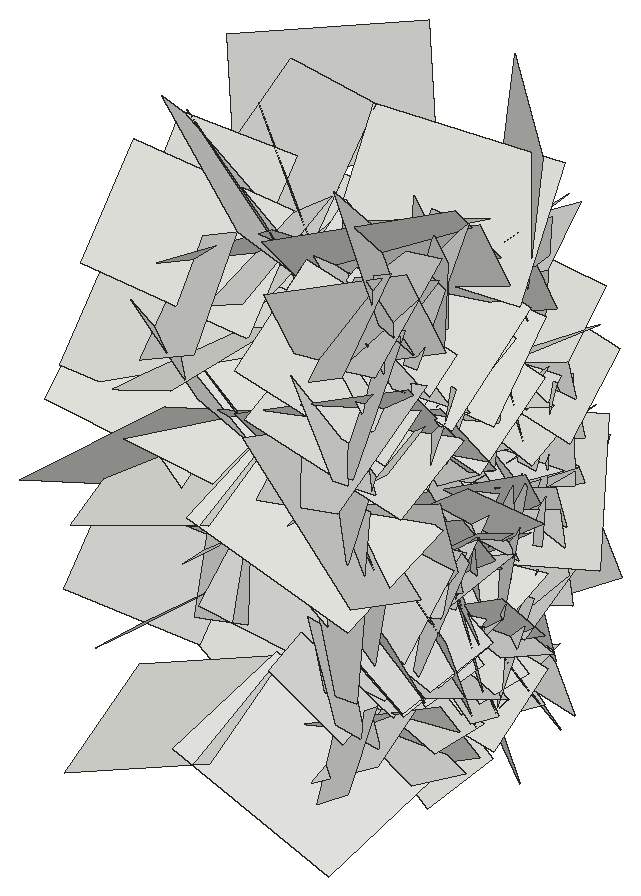
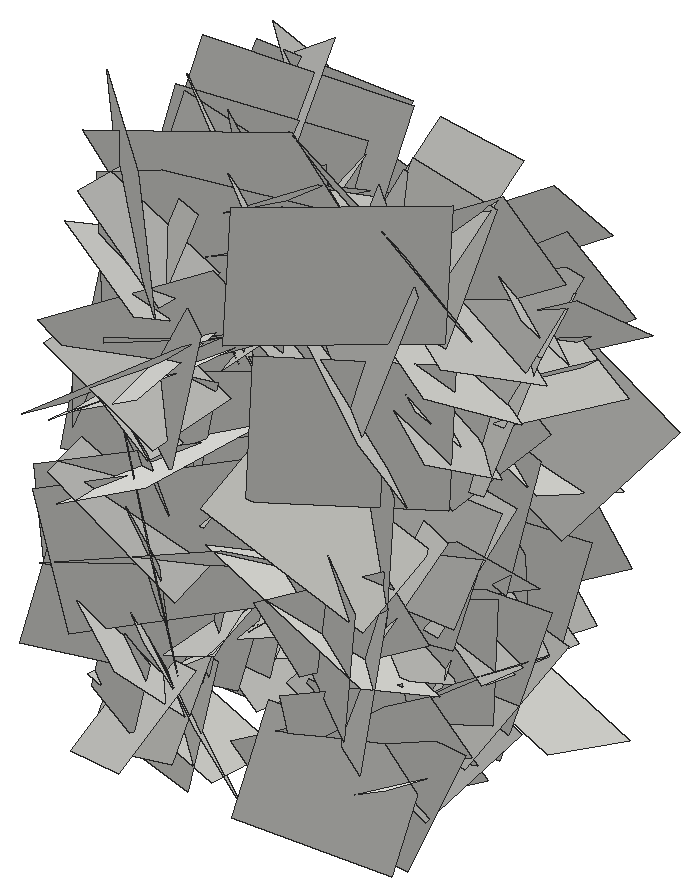
# SketchUp Ruby script. Lengths in inches.
U = 1.inch
M = Sketchup.active_model
def pt(a) = Geom::Point3d.new(a.map { |v| v * U })
def face(e, loops, mat)
  f = e.add_face(loops[0].map { |a| pt(a) })
  loops[1..].each { |l| e.add_face(l.map { |a| pt(a) }).erase! }
  f.material = f.back_material = mat if mat
  f
end
# faces: each face lists its corners as indices into pts; further lists are holes
def faces(e, pts, list, mat = nil) = list.each { |f| face(e, (f[0].is_a?(Array) ? f : [f]).map { |l| l.map { |i| pts[i] } }, mat) }
# xy, xz, yz: faces in a plane at the given z, y or x. An outline is a flat list of corners, or four numbers for a rectangle; further outlines are holes
def ring(l) = l.size == 4 ? [[l[0], l[1]], [l[2], l[1]], [l[2], l[3]], [l[0], l[3]]] : l.each_slice(2).to_a
def flat(e, list, mat, &to3) = list.each { |f| face(e, (f[0].is_a?(Array) ? f : [f]).map { |l| ring(l).map { |u, v| to3.(u, v) } }, mat) }
def xy(e, z, list, mat = nil) = flat(e, list, mat) { |x, y| [x, y, z] }
def xz(e, y, list, mat = nil) = flat(e, list, mat) { |x, z| [x, y, z] }
def yz(e, x, list, mat = nil) = flat(e, list, mat) { |y, z| [x, y, z] }
def lines(e, pts, list) = list.each { |a, b| e.add_line(pt(pts[a]), pt(pts[b])) }
# prism: a flat outline (further loops are holes) pulled along v
def prism(e, loops, v, mat = nil)
  f = face(e, loops, mat); d = Geom::Vector3d.new(v.map { |x| x * U })
  f.pushpull(f.normal.samedirection?(d) ? d.length : -d.length)
end
def box(e, o, s, mat = nil) = prism(e, [[o, [o[0] + s[0], o[1], o[2]], [o[0] + s[0], o[1] + s[1], o[2]], [o[0], o[1] + s[1], o[2]]]], [0, 0, s[2]], mat)
def at(x, y, z, deg = 0) = Geom::Transformation.translation(pt([x, y, z])) * Geom::Transformation.rotation(ORIGIN, Z_AXIS, deg.degrees)
def axes(o, x, y, z) = Geom::Transformation.new([*x, 0, *y, 0, *z, 0, *pt(o).to_a, 1])
def part(name) = M.definitions.add(name)
# library, detail: a bought-in or finely detailed component or shape, given as its bounding box
def library(name, o, s) = part(name).tap { |d| box(d.entities, o, s) }
def detail(e, o, s) = box(e.add_group.entities, o, s)
def put(e, d, t, mat = nil) = e.add_instance(d, t).tap { |i| i.material = mat if mat }
def group(e, t, mat = nil) = e.add_group.tap { |g| g.transformation = t; g.material = mat if mat }.entities
root = M.entities
c1 = part("Component\#6")
p = [[0.01,0,0],[0,3.24,4.54],[4.32,3.24,4.54],[4.33,0,0]]
faces(c1.entities,p,[[0,1,2,3]])
put(root,c1,axes([400.91,167.01,8.33],[0.18631,0.3359,0.73427],[0.04897,0.74605,-0.35235],[0.8545,-0.11599,-0.1399]))
put(root,c1,axes([400.91,166.18,19.56],[-0.12535,0.0531,1.28965],[-0.2192,1.27754,-0.07157],[1.35051,0.21229,0.10808]))
put(root,c1,axes([400.91,168.14,0.12],[-0.06773,-0.63363,0.78179],[0.11595,0.77435,0.63654],[1.06038,-0.12515,-0.01967]))
put(root,c1,axes([400.91,169.19,10.7],[-0.0913,0.46499,-1.24639],[-0.29576,-1.22753,-0.43867],[1.37875,-0.23253,-0.17663]))
put(root,c1,axes([404.88,165.96,10.85],[0.09912,0.20412,-0.70693],[0.02587,-0.71308,-0.20267],[-0.77953,0.00229,-0.09661]))
put(root,c1,axes([404.88,161.25,17.66],[0.25985,0.898,-0.37026],[0.14737,-0.41038,-0.90325],[-1.01902,0.16964,-0.22504]))
put(root,c1,axes([404.88,162.79,15.86],[0.07285,0.46729,0.4905],[-0.02436,0.49435,-0.46773],[-0.71769,0.03066,0.06566]))
put(root,c1,axes([400.91,167.22,15.375],[-0.0235,-0.92066,-0.53568],[-0.01768,-0.53543,0.92093],[1.12894,-0.02755,0.00327]))
put(root,c1,axes([400.91,167.28,17.92],[-0.19972,-0.96368,-0.57877],[0.14667,-0.60226,0.95775],[1.18251,-0.08806,-0.21655]))
put(root,c1,axes([400.91,157.18,19.73],[-0.07599,0.81527,0.8297],[-0.084,0.82592,-0.8184],[1.23014,0.10676,-0.00463]))
put(root,c1,axes([400.91,167.18,1.59],[-0.07507,-1.0991,0.32301],[-0.05871,0.32653,1.09895],[1.2129,-0.05222,0.07319]))
put(root,c1,axes([400.91,168.87,14.79],[0.03205,0.06087,-1.12787],[-0.16204,-1.11767,-0.06442],[1.18627,-0.15431,0.02167]))
put(root,c1,axes([400.91,166.01,11.8],[0.21466,0.53877,-0.68228],[-0.03009,-0.69607,-0.55809],[0.92102,-0.14831,0.14079]))
put(root,c1,axes([400.91,163.57,3.71],[0.11292,-0.2033,0.99476],[-0.09749,0.99417,0.21302],[1.07181,0.11185,-0.08542]))
put(root,c1,axes([400.91,159.91,9.22],[-0.2022,-1.20502,0.50539],[-0.1049,0.52261,1.20871],[1.38114,-0.13672,0.1658]))
put(root,c1,axes([400.91,162.44,14.8125],[-0.22172,-1.13603,-0.19278],[0.19013,-0.22565,1.13507],[1.20652,-0.17321,-0.21429]))
put(root,c1,axes([400.91,160.62,5.12],[0.08568,1.04485,0.18773],[-0.09569,0.19436,-1.04286],[1.1212,-0.06325,-0.10335]))
put(root,c1,axes([404.88,162.91,7.6875],[0.03517,0.6334,0.29771],[0.1292,0.28826,-0.62688],[-0.73053,0.08147,-0.09654]))
put(root,c1,axes([400.91,163.93,5.47],[0.11462,-1.01834,-0.26907],[-0.10191,-0.2789,1.0169],[1.11183,0.07941,0.12095]))
put(root,c1,axes([400.91,156.14,6.5],[0.17845,0.35117,0.84391],[0.01887,0.85668,-0.36003],[0.96872,-0.08137,-0.14844]))
put(root,c1,axes([404.88,170.02,6.34],[0.13634,-0.30577,-0.6303],[0.02329,-0.63876,0.31436],[-0.74222,-0.07621,-0.10592]))
put(root,c1,axes([400.91,160.14,4.78],[0.03826,-0.47304,0.81506],[0.18962,0.80427,0.45886],[0.98077,-0.13704,-0.12051]))
put(root,c1,axes([400.91,166.625,12.7],[0.17127,1.04033,-0.10676],[-0.13463,-0.08771,-1.04688],[1.10034,-0.17266,-0.11147]))
put(root,c1,axes([400.91,168.99,0.33],[0.20008,-0.71049,0.66963],[-0.07161,0.67089,0.73087],[1.03242,0.18422,-0.07908]))
put(root,c1,axes([400.91,164.18,5.53],[0.00871,-1.21515,-0.1589],[-0.11926,-0.15898,1.20995],[1.29354,-0.00648,0.11262]))
put(root,c1,axes([404.88,159.77,13.93],[0.14822,0.47929,0.38572],[-0.01533,0.39801,-0.48932],[-0.65196,0.0996,0.0992]))
put(root,c1,axes([400.91,165.6875,8.33],[0.14254,-0.77018,0.64298],[0.05856,0.65343,0.77114],[1.06187,0.06735,-0.12884]))
put(root,c1,axes([400.91,164.53,2.65],[0.11418,0.95876,0.15487],[0.16789,0.13639,-0.95453],[1.01568,-0.13033,0.14037]))
put(root,c1,axes([404.88,155.94,6.59],[0.14653,0.65267,0.04592],[0.0729,0.03218,-0.6644],[-0.6897,0.14207,-0.06047]))
put(root,c1,axes([400.91,170.79,17.67],[0.07972,-0.69903,-0.88266],[-0.01234,-0.88506,0.69994],[1.19343,0.03754,0.0662]))
put(root,c1,axes([400.91,165.97,13.03],[0.11695,-0.23373,1.15092],[-0.10796,1.14973,0.24325],[1.24018,0.12213,-0.08736]))
put(root,c1,axes([404.88,164.09,3.1],[0.16189,-0.51758,0.36968],[0.06161,0.38995,0.52196],[-0.67139,-0.08902,0.13704]))
put(root,c1,axes([400.91,155.93,16.01],[0.06166,0.77521,1.08886],[-0.24821,1.07895,-0.75564],[1.39492,0.15772,-0.18259]))
put(root,c1,axes([400.91,163.21,2.24],[-0.08398,-0.53221,1.10764],[0.11648,1.10243,0.53756],[1.29738,-0.13342,0.02343]))
put(root,c1,axes([400.91,161.02,12.77],[0.04866,0.36936,-1.04237],[0.12613,-1.03886,-0.36288],[1.16543,0.09701,0.0828]))
put(root,c1,axes([400.91,162.03,18.62],[0.15865,-0.78055,-0.79386],[-0.03617,-0.80384,0.78393],[1.17956,0.08034,0.13081]))
put(root,c1,axes([400.91,161.03,16.77],[-0.02327,0.73455,-0.90907],[0.17416,-0.89826,-0.72978],[1.22657,0.14148,0.08637]))
put(root,c1,axes([400.91,163.86,1.73],[0.03729,0.66749,1.03354],[-0.00972,1.03407,-0.66752],[1.30413,-0.01138,-0.03452]))
put(root,c1,axes([400.91,162.85,15.75],[0.04254,-1.00522,0.67204],[0.02385,0.67292,1.00519],[1.28151,0.02084,-0.04102]))
put(root,c1,axes([400.91,163.36,23.49],[0.04873,0.57368,-1.00395],[0.12423,-1.00188,-0.56714],[1.21936,0.07915,0.09791]))
put(root,c1,axes([400.91,159.69,18.96],[0.02704,0.74145,1.09535],[-0.09362,1.09406,-0.73853],[1.39894,0.05888,-0.07059]))
put(root,c1,axes([400.91,166.4,18.65],[-0.092,-1.19571,-0.63762],[0.0325,-0.6405,1.19693],[1.43603,-0.06211,-0.06794]))
put(root,c1,axes([400.91,155.03,14.95],[-0.10989,1.07322,0.82249],[0.07177,0.82799,-1.07186],[1.43147,0.04087,0.11688]))
put(root,c1,axes([400.91,159.14,18.38],[0.07521,0.79304,-0.86536],[0.12573,-0.86735,-0.78513],[1.23784,0.03991,0.13233]))
put(root,c1,axes([400.91,168.375,23.9],[-0.0952,-0.72561,-1.04974],[0.29336,-1.03837,0.69407],[1.32049,0.17837,-0.22987]))
put(root,c1,axes([400.91,157.93,15.34],[0.27083,1.19165,0.15594],[-0.0802,0.17506,-1.21378],[1.27139,-0.2428,-0.10978]))
put(root,c1,axes([400.91,162.31,11.53],[0.17206,0.75955,-0.87532],[0.12131,-0.89005,-0.75111],[1.22246,-0.01858,0.19774]))
put(root,c1,axes([400.91,165.1,2.71],[-0.06092,-1.21711,0.58199],[0.18306,0.57109,1.21136],[1.41828,-0.12599,-0.13136]))
put(root,c1,axes([400.91,170.58,10.37],[0.24309,-1.14649,0.14454],[0.04952,0.15643,1.16674],[1.2239,0.22139,-0.07591]))
put(root,c1,axes([400.91,161.07,7.88],[0.0926,0.91308,0.78861],[0.24837,0.76278,-0.90913],[1.25453,-0.21841,0.12178]))
put(root,c1,axes([400.91,171.01,11.29],[0.23144,-0.15428,-1.27652],[-0.01824,-1.29503,0.15357],[1.36284,0.00887,0.21884]))
put(root,c1,axes([400.91,167.61,21.95],[0.32344,0.31012,-1.26322],[-0.1451,-1.28265,-0.34796],[1.37111,-0.2089,0.26116]))
put(root,c1,axes([400.91,161.91,24.73],[0.20116,0.87735,-0.9177],[0.06395,-0.93308,-0.87958],[1.34427,-0.0869,0.17917]))
put(root,c1,axes([400.91,161.24,11.55],[0.08722,-1.18104,-0.51149],[0.30261,-0.48302,1.16122],[1.33028,0.18731,-0.23062]))
put(root,c1,axes([400.91,160.65,1.35],[0.1594,-1.22011,-0.46707],[0.28659,-0.43091,1.2127],[1.35486,0.2347,-0.20157]))
put(root,c1,axes([400.91,170.67,8.29],[0.13658,-1.14766,-0.62909],[0.33753,-0.58565,1.13362],[1.34561,0.26339,-0.2205]))
put(root,c1,axes([400.91,161.87,9.58],[0.35888,-0.49511,-1.17449],[0.11741,-1.19919,0.53746],[1.34594,0.23663,0.26628]))
put(root,c1,axes([414.68,161.87,9.58],[-0.35888,-0.49511,-1.17449],[-0.11741,-1.19919,0.53746],[-1.34594,0.23663,0.26628]))
put(root,c1,axes([414.68,170.67,8.29],[-0.13658,-1.14766,-0.62909],[-0.33753,-0.58565,1.13362],[-1.34561,0.26339,-0.2205]))
put(root,c1,axes([414.68,160.65,1.35],[-0.1594,-1.22011,-0.46707],[-0.28659,-0.43091,1.2127],[-1.35486,0.2347,-0.20157]))
put(root,c1,axes([414.68,161.24,11.55],[-0.08722,-1.18104,-0.51149],[-0.30261,-0.48302,1.16122],[-1.33028,0.18731,-0.23062]))
put(root,c1,axes([414.68,161.91,24.73],[-0.20116,0.87735,-0.9177],[-0.06395,-0.93308,-0.87958],[-1.34427,-0.0869,0.17917]))
put(root,c1,axes([414.68,167.61,21.95],[-0.32344,0.31012,-1.26322],[0.1451,-1.28265,-0.34796],[-1.37111,-0.2089,0.26116]))
put(root,c1,axes([414.68,171.01,11.29],[-0.23144,-0.15428,-1.27652],[0.01824,-1.29503,0.15357],[-1.36284,0.00887,0.21884]))
put(root,c1,axes([414.68,161.07,7.88],[-0.0926,0.91308,0.78861],[-0.24837,0.76278,-0.90913],[-1.25453,-0.21841,0.12178]))
put(root,c1,axes([414.68,170.58,10.37],[-0.24309,-1.14649,0.14454],[-0.04952,0.15643,1.16674],[-1.2239,0.22139,-0.07591]))
put(root,c1,axes([414.68,165.1,2.71],[0.06092,-1.21711,0.58199],[-0.18306,0.57109,1.21136],[-1.41828,-0.12599,-0.13136]))
put(root,c1,axes([414.68,162.31,11.53],[-0.17206,0.75955,-0.87532],[-0.12131,-0.89005,-0.75111],[-1.22246,-0.01858,0.19774]))
put(root,c1,axes([414.68,157.93,15.34],[-0.27083,1.19165,0.15594],[0.0802,0.17506,-1.21378],[-1.27139,-0.2428,-0.10978]))
put(root,c1,axes([414.68,168.375,23.9],[0.0952,-0.72561,-1.04974],[-0.29336,-1.03837,0.69407],[-1.32049,0.17837,-0.22987]))
put(root,c1,axes([414.68,159.14,18.38],[-0.07521,0.79304,-0.86536],[-0.12573,-0.86735,-0.78513],[-1.23784,0.03991,0.13233]))
put(root,c1,axes([414.68,155.03,14.95],[0.10989,1.07322,0.82249],[-0.07177,0.82799,-1.07186],[-1.43147,0.04087,0.11688]))
put(root,c1,axes([414.68,166.4,18.65],[0.092,-1.19571,-0.63762],[-0.0325,-0.6405,1.19693],[-1.43603,-0.06211,-0.06794]))
put(root,c1,axes([414.68,159.69,18.96],[-0.02704,0.74145,1.09535],[0.09362,1.09406,-0.73853],[-1.39894,0.05888,-0.07059]))
put(root,c1,axes([414.68,163.36,23.49],[-0.04873,0.57368,-1.00395],[-0.12423,-1.00188,-0.56714],[-1.21936,0.07915,0.09791]))
put(root,c1,axes([414.68,162.85,15.75],[-0.04254,-1.00522,0.67204],[-0.02385,0.67292,1.00519],[-1.28151,0.02084,-0.04102]))
put(root,c1,axes([414.68,163.86,1.73],[-0.03729,0.66749,1.03354],[0.00972,1.03407,-0.66752],[-1.30413,-0.01138,-0.03452]))
put(root,c1,axes([414.68,161.03,16.77],[0.02327,0.73455,-0.90907],[-0.17416,-0.89826,-0.72978],[-1.22657,0.14148,0.08637]))
put(root,c1,axes([414.68,162.03,18.62],[-0.15865,-0.78055,-0.79386],[0.03617,-0.80384,0.78393],[-1.17956,0.08034,0.13081]))
put(root,c1,axes([414.68,161.02,12.77],[-0.04866,0.36936,-1.04237],[-0.12613,-1.03886,-0.36288],[-1.16543,0.09701,0.0828]))
put(root,c1,axes([414.68,163.21,2.24],[0.08398,-0.53221,1.10764],[-0.11648,1.10243,0.53756],[-1.29738,-0.13342,0.02343]))
put(root,c1,axes([414.68,155.93,16.01],[-0.06166,0.77521,1.08886],[0.24821,1.07895,-0.75564],[-1.39492,0.15772,-0.18259]))
put(root,c1,axes([410.71,164.09,3.1],[-0.16189,-0.51758,0.36968],[-0.06161,0.38995,0.52196],[0.67139,-0.08902,0.13704]))
put(root,c1,axes([414.68,165.97,13.03],[-0.11695,-0.23373,1.15092],[0.10796,1.14973,0.24325],[-1.24018,0.12213,-0.08736]))
put(root,c1,axes([414.68,170.79,17.67],[-0.07972,-0.69903,-0.88266],[0.01234,-0.88506,0.69994],[-1.19343,0.03754,0.0662]))
put(root,c1,axes([410.71,155.94,6.59],[-0.14653,0.65267,0.04592],[-0.0729,0.03218,-0.6644],[0.6897,0.14207,-0.06047]))
put(root,c1,axes([414.68,164.53,2.65],[-0.11418,0.95876,0.15487],[-0.16789,0.13639,-0.95453],[-1.01568,-0.13033,0.14037]))
put(root,c1,axes([414.68,165.6875,8.33],[-0.14254,-0.77018,0.64298],[-0.05856,0.65343,0.77114],[-1.06187,0.06735,-0.12884]))
put(root,c1,axes([410.71,159.77,13.93],[-0.14822,0.47929,0.38572],[0.01533,0.39801,-0.48932],[0.65196,0.0996,0.0992]))
put(root,c1,axes([414.68,164.18,5.53],[-0.00871,-1.21515,-0.1589],[0.11926,-0.15898,1.20995],[-1.29354,-0.00648,0.11262]))
put(root,c1,axes([414.68,168.99,0.33],[-0.20008,-0.71049,0.66963],[0.07161,0.67089,0.73087],[-1.03242,0.18422,-0.07908]))
put(root,c1,axes([414.68,166.625,12.7],[-0.17127,1.04033,-0.10676],[0.13463,-0.08771,-1.04688],[-1.10034,-0.17266,-0.11147]))
put(root,c1,axes([414.68,160.14,4.78],[-0.03826,-0.47304,0.81506],[-0.18962,0.80427,0.45886],[-0.98077,-0.13704,-0.12051]))
put(root,c1,axes([410.71,170.02,6.34],[-0.13634,-0.30577,-0.6303],[-0.02329,-0.63876,0.31436],[0.74222,-0.07621,-0.10592]))
put(root,c1,axes([414.68,156.14,6.5],[-0.17845,0.35117,0.84391],[-0.01887,0.85668,-0.36003],[-0.96872,-0.08137,-0.14844]))
put(root,c1,axes([414.68,163.93,5.47],[-0.11462,-1.01834,-0.26907],[0.10191,-0.2789,1.0169],[-1.11183,0.07941,0.12095]))
put(root,c1,axes([410.71,162.91,7.6875],[-0.03517,0.6334,0.29771],[-0.1292,0.28826,-0.62688],[0.73053,0.08147,-0.09654]))
put(root,c1,axes([414.68,160.62,5.12],[-0.08568,1.04485,0.18773],[0.09569,0.19436,-1.04286],[-1.1212,-0.06325,-0.10335]))
put(root,c1,axes([414.68,162.44,14.8125],[0.22172,-1.13603,-0.19278],[-0.19013,-0.22565,1.13507],[-1.20652,-0.17321,-0.21429]))
put(root,c1,axes([414.68,159.91,9.22],[0.2022,-1.20502,0.50539],[0.1049,0.52261,1.20871],[-1.38114,-0.13672,0.1658]))
put(root,c1,axes([414.68,163.57,3.71],[-0.11292,-0.2033,0.99476],[0.09749,0.99417,0.21302],[-1.07181,0.11185,-0.08542]))
put(root,c1,axes([414.68,166.01,11.8],[-0.21466,0.53877,-0.68228],[0.03009,-0.69607,-0.55809],[-0.92102,-0.14831,0.14079]))
put(root,c1,axes([414.68,168.87,14.79],[-0.03205,0.06087,-1.12787],[0.16204,-1.11767,-0.06442],[-1.18627,-0.15431,0.02167]))
put(root,c1,axes([414.68,167.18,1.59],[0.07507,-1.0991,0.32301],[0.05871,0.32653,1.09895],[-1.2129,-0.05222,0.07319]))
put(root,c1,axes([414.68,157.18,19.73],[0.07599,0.81527,0.8297],[0.084,0.82592,-0.8184],[-1.23014,0.10676,-0.00463]))
put(root,c1,axes([414.68,167.28,17.92],[0.19972,-0.96368,-0.57877],[-0.14667,-0.60226,0.95775],[-1.18251,-0.08806,-0.21655]))
put(root,c1,axes([414.68,167.22,15.375],[0.0235,-0.92066,-0.53568],[0.01768,-0.53543,0.92093],[-1.12894,-0.02755,0.00327]))
put(root,c1,axes([410.71,162.79,15.86],[-0.07285,0.46729,0.4905],[0.02436,0.49435,-0.46773],[0.71769,0.03066,0.06566]))
put(root,c1,axes([410.71,161.25,17.66],[-0.25985,0.898,-0.37026],[-0.14737,-0.41038,-0.90325],[1.01902,0.16964,-0.22504]))
put(root,c1,axes([410.71,165.96,10.85],[-0.09912,0.20412,-0.70693],[-0.02587,-0.71308,-0.20267],[0.77953,0.00229,-0.09661]))
put(root,c1,axes([414.68,169.19,10.7],[0.0913,0.46499,-1.24639],[0.29576,-1.22753,-0.43867],[-1.37875,-0.23253,-0.17663]))
put(root,c1,axes([414.68,168.14,0.12],[0.06773,-0.63363,0.78179],[-0.11595,0.77435,0.63654],[-1.06038,-0.12515,-0.01967]))
put(root,c1,axes([414.68,166.18,19.56],[0.12535,0.0531,1.28965],[0.2192,1.27754,-0.07157],[-1.35051,0.21229,0.10808]))
put(root,c1,axes([414.68,167.01,8.33],[-0.18631,0.3359,0.73427],[-0.04897,0.74605,-0.35235],[-0.8545,-0.11599,-0.1399]))
put(root,c1,axes([410.71,159.82,10.86],[-0.164,0.05549,-0.7166],[0.119,-0.72215,-0.08015],[0.75252,0.12629,-0.14349]))
put(root,c1,axes([414.68,164.72,6.23],[0.02586,0.29335,1.1723],[0.23754,1.1511,-0.29271],[-1.25874,0.22326,-0.03115]))
put(root,c1,axes([410.71,164.71,11.17],[-0.09162,-0.23701,0.75882],[-0.09076,0.76162,0.22813],[0.83777,0.05659,0.1077]))
put(root,c1,axes([410.71,167.39,12.19],[-0.06725,0.11282,-0.6237],[0.12717,-0.61335,-0.12315],[0.65971,0.12973,-0.03984]))
put(root,c1,axes([410.71,158.25,7.85],[0.01053,0.60228,-0.51533],[-0.19634,-0.49934,-0.58716],[0.81696,-0.12777,-0.13447]))
put(root,c1,axes([414.68,165.51,17.74],[-0.00528,-0.97827,-0.44464],[0.11526,-0.44282,0.97306],[-1.13321,-0.04048,0.10104]))
put(root,c1,axes([414.68,165.75,-1.09],[0.03685,-0.4153,0.96157],[0.02645,0.96216,0.41465],[-1.10996,0.00914,0.04181]))
put(root,c1,axes([414.68,167.74,3.51],[0.11337,-0.86322,0.3774],[-0.28126,0.33685,0.84566],[-0.95821,-0.201,-0.20357]))
put(root,c1,axes([414.68,161.03,4.22],[-0.00206,0.54706,-0.73945],[-0.10036,-0.73565,-0.544],[-0.96983,0.07497,0.05787]))
put(root,c1,axes([414.68,158.84,13.7],[-0.15038,-0.75335,0.50607],[0.08727,0.49942,0.76653],[-0.95804,0.16374,-0.00961]))
put(root,c1,axes([414.68,166.72,20.27],[-0.14718,0.45385,-0.66356],[-0.05291,-0.67695,-0.45256],[-0.85051,-0.03642,0.14299]))
put(root,c1,axes([410.71,158.82,19.64],[0.09205,0.73549,-0.019],[-0.17536,0.00088,-0.72213],[0.75991,-0.08889,-0.16434]))
put(root,c1,axes([414.68,169.09,13.37],[-0.12805,-0.81492,0.2825],[0.01832,0.28292,0.8235],[-0.91406,0.11983,-0.02307]))
put(root,c1,axes([410.71,159.61,12.59],[0.0897,0.16152,-0.57424],[0.01993,-0.58042,-0.16049],[0.632,-0.00462,0.08656]))
put(root,c1,axes([410.71,160.65,18.69],[0.1336,-0.1743,0.59472],[-0.06624,0.60023,0.18916],[0.65357,0.09646,-0.1024]))
put(root,c1,axes([410.71,160.54,14.42],[-0.065,-0.29459,-0.75204],[-0.0763,-0.74921,0.29935],[0.85274,-0.0895,-0.03054]))
put(root,c1,axes([410.71,161.26,10.83],[-0.08958,0.45503,-0.59155],[0.06652,-0.58889,-0.46195],[0.78829,0.10141,-0.02824]))
put(root,c1,axes([414.68,170.16,13.55],[0.14984,-1.04824,-0.22204],[-0.00627,-0.22472,1.05715],[-1.13577,-0.13705,-0.03513]))
put(root,c1,axes([410.71,160.97,6.7],[0.04912,0.73058,0.10133],[-0.09877,0.10652,-0.72536],[0.77557,-0.03271,-0.0988]))
put(root,c1,axes([414.68,163.26,10.51],[-0.09772,0.8385,-0.3881],[0.10419,-0.37892,-0.842],[-0.97385,-0.12468,-0.05114]))
put(root,c1,axes([410.71,159.79,25.07],[-0.1328,0.69586,-0.68383],[-0.18687,-0.69425,-0.67416],[1.01714,-0.03669,-0.21313]))
put(root,c1,axes([414.68,167.39,3.05],[0.22625,-1.02118,-0.283],[-0.12014,-0.30902,1.02962],[-1.11681,-0.17363,-0.16809]))
put(root,c1,axes([410.71,159.32,12.84],[0.06752,-0.16321,-0.59207],[0.0871,-0.58763,0.17083],[0.64514,0.09641,0.0389]))
put(root,c1,axes([410.71,169.73,5.36],[0.07377,0.11031,-0.61615],[0.06228,-0.61836,-0.10407],[0.66058,0.04598,0.07863]))
put(root,c1,axes([414.68,166.22,16.78],[0.0558,0.90138,-0.08554],[-0.09664,-0.07998,-0.89882],[-0.95488,0.06076,0.08597]))
put(root,c1,axes([410.71,166.8,6.58],[-0.19077,-0.84984,-0.315],[0.00737,-0.32244,0.86593],[0.9607,-0.16629,-0.0692]))
put(root,c1,axes([414.68,159.03,23.29],[0.13252,0.38295,-0.87838],[-0.10893,-0.87536,-0.39626],[-1.00987,0.14467,-0.07253]))
put(root,c1,axes([410.71,160.57,3.12],[0.03509,0.82869,0.13415],[-0.15764,0.13792,-0.81528],[0.87577,-0.00838,-0.15213]))
put(root,c1,axes([410.71,164.04,15.7],[0.03624,-0.6234,-0.24842],[0.08,-0.24359,0.62167],[0.70683,0.05954,-0.05762]))
put(root,c1,axes([414.68,170.98,12.21],[0.31631,-0.51758,-1.19288],[0.16648,-1.20059,0.56021],[-1.36826,-0.26573,-0.20761]))
put(root,c1,axes([410.71,169.83,13.22],[0.13817,-0.64015,-0.16037],[-0.03989,-0.17041,0.64965],[0.69839,0.11692,0.06883]))
put(root,c1,axes([410.71,161.46,7.67],[0.11157,-0.00104,0.59962],[0.09459,0.60203,-0.01462],[0.62852,-0.09042,-0.10424]))
put(root,c1,axes([414.68,168.08,9.41],[0.11593,0.02752,-0.90523],[-0.14705,-0.90054,-0.04413],[-0.94866,0.14295,-0.10378]))
put(root,c1,axes([410.71,169.26,18.83],[0.02849,-0.83115,-0.05333],[-0.13283,-0.05679,0.82186],[0.87278,0.01849,0.12683]))
put(root,c1,axes([410.71,165.55,15.88],[-0.02597,-0.35934,-0.67832],[0.02345,-0.67872,0.35875],[0.81334,0.00809,-0.032]))
put(root,c1,axes([410.71,167.12,21.5],[0.0656,0.35319,-0.61189],[0.00255,-0.61434,-0.35436],[0.7489,-0.02885,0.0548]))
put(root,c1,axes([414.68,164.04,2.37],[0.08884,-0.86849,0.07962],[-0.14736,0.06566,0.86256],[-0.91264,-0.09515,-0.13152]))
put(root,c1,axes([414.68,162.54,0.74],[0.05881,-0.79857,0.25436],[-0.14334,0.24305,0.79255],[-0.87675,-0.0933,-0.11251]))
put(root,c1,axes([414.68,157.37,3.29],[-0.12325,0.67494,0.21472],[-0.06797,0.20667,-0.68436],[-0.74769,-0.13004,0.02682]))
put(root,c1,axes([414.68,166.02,4.84],[0.16866,0.71959,0.68076],[-0.0323,0.69272,-0.72511],[-1.04952,0.09433,0.13172]))
put(root,c1,axes([410.71,162.4,12.14],[0.15913,-0.1111,0.71617],[-0.10617,0.72117,0.13287],[0.76084,0.12387,-0.13124]))
put(root,c1,axes([410.71,165.06,16.01],[-0.24936,0.99659,0.4051],[-0.07669,0.39908,-1.02378],[1.13774,0.24532,0.01978]))
put(root,c1,axes([410.71,164.7,6.68],[-0.19863,-0.78204,0.62344],[-0.03401,0.63866,0.7915],[1.0596,-0.1261,0.14227]))
put(root,c1,axes([414.68,166.67,11.65],[-0.03639,0.32382,0.70516],[-0.0632,0.70266,-0.32558],[-0.82009,-0.06852,-0.0062]))
put(root,c1,axes([414.68,166.25,3.34],[-0.10377,-0.78092,-0.09398],[0.04515,-0.09983,0.78516],[-0.83253,0.09192,0.05429]))
put(root,c1,axes([414.68,167.84,10.46],[0.01526,0.23241,-0.73689],[-0.14958,-0.72384,-0.23105],[-0.80526,0.13886,0.02896]))
put(root,c1,axes([414.68,164.66,7.18],[0.03191,0.54978,-0.59147],[-0.106,-0.58478,-0.54866],[-0.84939,0.09364,0.04625]))
put(root,c1,axes([414.68,155.24,20.59],[-0.01301,0.69003,0.71111],[0.211,0.69839,-0.67424],[-1.02891,0.13449,-0.14726]))
put(root,c1,axes([414.68,167.39,19.82],[-0.12929,0.6108,0.35138],[-0.02449,0.35295,-0.62154],[-0.74654,-0.11736,-0.04046]))
put(root,c1,axes([410.71,165.07,9.38],[0.13081,0.27606,-0.70722],[-0.08788,-0.70731,-0.29057],[0.79993,-0.12284,0.08373]))
put(root,c1,axes([414.68,159.79,6],[0.13547,0.51146,0.93772],[0.15367,0.92736,-0.52557],[-1.12174,0.18881,0.04125]))
put(root,c1,axes([414.68,159.9,13.67],[0.02397,0.44215,0.82689],[0.11898,0.8199,-0.44149],[-0.98679,0.1096,-0.03314]))
put(root,c1,axes([410.71,164.44,22.83],[-0.02931,-0.02413,-0.88007],[-0.04764,-0.87932,0.02552],[0.93201,-0.0457,-0.02637]))
put(root,c1,axes([414.68,168.54,15.47],[0.051,0.16682,-0.79913],[-0.09039,-0.79511,-0.17112],[-0.86061,0.0934,-0.02938]))
put(root,c1,axes([414.68,155.625,2.89],[-0.13104,0.56412,0.5606],[0.11872,0.57403,-0.55293],[-0.83462,-0.00692,-0.16667]))
